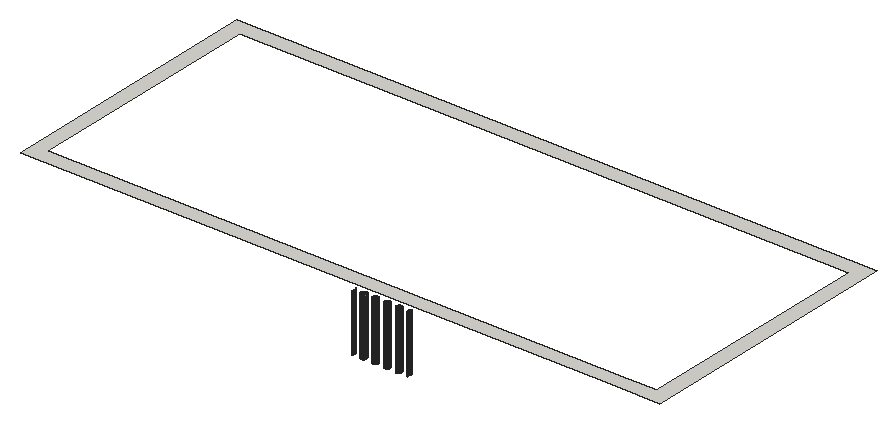
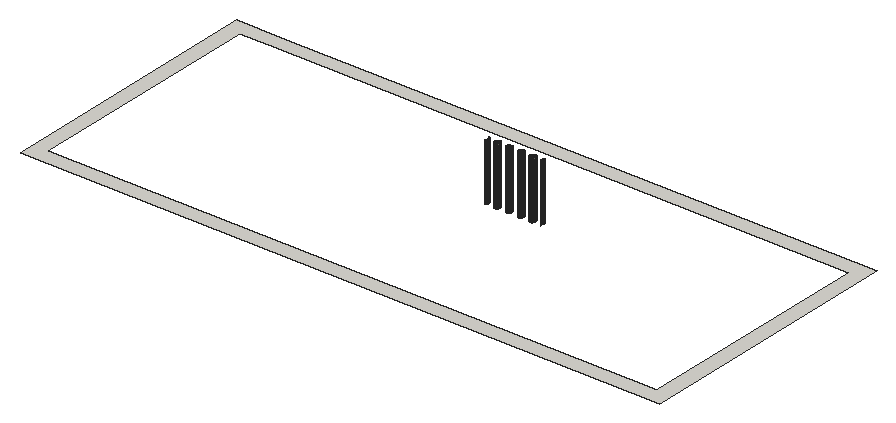
# SketchUp Ruby script. Lengths in inches.
U = 1.inch
M = Sketchup.active_model
def pt(a) = Geom::Point3d.new(a.map { |v| v * U })
def face(e, loops, mat)
  f = e.add_face(loops[0].map { |a| pt(a) })
  loops[1..].each { |l| e.add_face(l.map { |a| pt(a) }).erase! }
  f.material = f.back_material = mat if mat
  f
end
# faces: each face lists its corners as indices into pts; further lists are holes
def faces(e, pts, list, mat = nil) = list.each { |f| face(e, (f[0].is_a?(Array) ? f : [f]).map { |l| l.map { |i| pts[i] } }, mat) }
# xy, xz, yz: faces in a plane at the given z, y or x. An outline is a flat list of corners, or four numbers for a rectangle; further outlines are holes
def ring(l) = l.size == 4 ? [[l[0], l[1]], [l[2], l[1]], [l[2], l[3]], [l[0], l[3]]] : l.each_slice(2).to_a
def flat(e, list, mat, &to3) = list.each { |f| face(e, (f[0].is_a?(Array) ? f : [f]).map { |l| ring(l).map { |u, v| to3.(u, v) } }, mat) }
def xy(e, z, list, mat = nil) = flat(e, list, mat) { |x, y| [x, y, z] }
def xz(e, y, list, mat = nil) = flat(e, list, mat) { |x, z| [x, y, z] }
def yz(e, x, list, mat = nil) = flat(e, list, mat) { |y, z| [x, y, z] }
def lines(e, pts, list) = list.each { |a, b| e.add_line(pt(pts[a]), pt(pts[b])) }
# prism: a flat outline (further loops are holes) pulled along v
def prism(e, loops, v, mat = nil)
  f = face(e, loops, mat); d = Geom::Vector3d.new(v.map { |x| x * U })
  f.pushpull(f.normal.samedirection?(d) ? d.length : -d.length)
end
def box(e, o, s, mat = nil) = prism(e, [[o, [o[0] + s[0], o[1], o[2]], [o[0] + s[0], o[1] + s[1], o[2]], [o[0], o[1] + s[1], o[2]]]], [0, 0, s[2]], mat)
def at(x, y, z, deg = 0) = Geom::Transformation.translation(pt([x, y, z])) * Geom::Transformation.rotation(ORIGIN, Z_AXIS, deg.degrees)
def axes(o, x, y, z) = Geom::Transformation.new([*x, 0, *y, 0, *z, 0, *pt(o).to_a, 1])
def part(name) = M.definitions.add(name)
# library, detail: a bought-in or finely detailed component or shape, given as its bounding box
def library(name, o, s) = part(name).tap { |d| box(d.entities, o, s) }
def detail(e, o, s) = box(e.add_group.entities, o, s)
def put(e, d, t, mat = nil) = e.add_instance(d, t).tap { |i| i.material = mat if mat }
def group(e, t, mat = nil) = e.add_group.tap { |g| g.transformation = t; g.material = mat if mat }.entities
root = M.entities
M.materials.add("[Formica Graystone]").color = [149, 146, 135]
M.materials.add("[Terrazzo Tile Light]").color = [219, 217, 210]
xy(root,552.75,[[326.25,21.93,325.54,22.02,324.875,22.3,324.31,22.74,323.87,23.3,323.59,23.97,323.5,24.68,323.59,25.39,323.87,26.05,324.31,26.625,324.875,27.0625,325.54,27.34,326.25,27.43,326.96,27.34,327.625,27.0625,328.19,26.625,328.63,26.05,328.91,25.39,329,24.68,328.91,23.97,328.63,23.3,328.19,22.74,327.625,22.3,326.96,22.02],[337.625,21.93,336.91,22.02,336.25,22.3,335.68,22.74,335.24,23.3,334.97,23.97,334.875,24.68,334.97,25.39,335.24,26.05,335.68,26.625,336.25,27.0625,336.91,27.34,337.625,27.43,338.34,27.34,339,27.0625,339.57,26.625,340.01,26.05,340.28,25.39,340.375,24.68,340.28,23.97,340.01,23.3,339.57,22.74,339,22.3,338.34,22.02],[349,21.93,348.29,22.02,347.625,22.3,347.06,22.74,346.62,23.3,346.34,23.97,346.25,24.68,346.34,25.39,346.62,26.05,347.06,26.625,347.625,27.0625,348.29,27.34,349,27.43,349.71,27.34,350.375,27.0625,350.94,26.625,351.38,26.05,351.66,25.39,351.75,24.68,351.66,23.97,351.38,23.3,350.94,22.74,350.375,22.3,349.71,22.02],[360.375,21.93,359.66,22.02,359,22.3,358.43,22.74,357.99,23.3,357.72,23.97,357.625,24.68,357.72,25.39,357.99,26.05,358.43,26.625,359,27.0625,359.66,27.34,360.375,27.43,361.09,27.34,361.75,27.0625,362.32,26.625,362.76,26.05,363.03,25.39,363.125,24.68,363.03,23.97,362.76,23.3,362.32,22.74,361.75,22.3,361.09,22.02]])
xy(root,619.9375,[[0,16.1875,577.38,16.1875,577.38,31.11,14.92,31.11,14.92,263.56,605.2,263.56,605.2,31.11,577.38,31.11,577.38,16.1875,620.12,16.1875,620.12,278.48,0,278.48]],"[Terrazzo Tile Light]")
p = [[325.54,22.02,552.75],[326.25,21.93,552.75],[326.25,21.93,608.75],[325.54,22.02,608.75],[326.96,22.02,552.75],[326.96,22.02,608.75],
  [336.91,22.02,552.75],[337.625,21.93,552.75],[337.625,21.93,608.75],[336.91,22.02,608.75],[338.34,22.02,552.75],[338.34,22.02,608.75],
  [348.29,22.02,552.75],[349,21.93,552.75],[349,21.93,608.75],[348.29,22.02,608.75],[349.71,22.02,552.75],[349.71,22.02,608.75],
  [359.66,22.02,552.75],[360.375,21.93,552.75],[360.375,21.93,608.75],[359.66,22.02,608.75],[361.09,22.02,552.75],[361.09,22.02,608.75],
  [324.875,22.3,552.75],[324.875,22.3,608.75],[327.625,22.3,552.75],[327.625,22.3,608.75],[336.25,22.3,552.75],[336.25,22.3,608.75],
  [339,22.3,552.75],[339,22.3,608.75],[347.625,22.3,552.75],[347.625,22.3,608.75],[350.375,22.3,552.75],[350.375,22.3,608.75],
  [359,22.3,552.75],[359,22.3,608.75],[361.75,22.3,552.75],[361.75,22.3,608.75],[370.375,22.3,552.75],[371.04,22.02,552.75],
  [371.04,22.02,608.75],[370.375,22.3,608.75],[316.25,22.3,552.75],[316.82,22.74,552.75],[316.82,22.74,608.75],[316.25,22.3,608.75],
  [324.31,22.74,552.75],[324.31,22.74,608.75],[328.19,22.74,552.75],[328.19,22.74,608.75],[335.68,22.74,552.75],[335.68,22.74,608.75],
  [339.57,22.74,552.75],[339.57,22.74,608.75],[347.06,22.74,552.75],[347.06,22.74,608.75],[350.94,22.74,552.75],[350.94,22.74,608.75],
  [358.43,22.74,552.75],[358.43,22.74,608.75],[362.32,22.74,552.75],[362.32,22.74,608.75],[369.81,22.74,552.75],[369.81,22.74,608.75],
  [317.26,23.3,552.75],[317.26,23.3,608.75],[323.87,23.3,552.75],[323.87,23.3,608.75],[328.63,23.3,552.75],[328.63,23.3,608.75],
  [335.24,23.3,552.75],[335.24,23.3,608.75],[340.01,23.3,552.75],[340.01,23.3,608.75],[346.62,23.3,552.75],[346.62,23.3,608.75],
  [351.38,23.3,552.75],[351.38,23.3,608.75],[357.99,23.3,552.75],[357.99,23.3,608.75],[362.76,23.3,552.75],[362.76,23.3,608.75],
  [369.37,23.3,552.75],[369.37,23.3,608.75],[317.53,23.97,552.75],[317.53,23.97,608.75],[323.59,23.97,552.75],[323.59,23.97,608.75],
  [328.91,23.97,552.75],[328.91,23.97,608.75],[334.97,23.97,552.75],[334.97,23.97,608.75],[340.28,23.97,552.75],[340.28,23.97,608.75],
  [346.34,23.97,552.75],[346.34,23.97,608.75],[351.66,23.97,552.75],[351.66,23.97,608.75],[357.72,23.97,552.75],[357.72,23.97,608.75],
  [363.03,23.97,552.75],[363.03,23.97,608.75],[369.09,23.97,552.75],[369.09,23.97,608.75],[317.625,24.68,552.75],[317.625,24.68,608.75],
  [323.5,24.68,552.75],[323.5,24.68,608.75],[329,24.68,552.75],[329,24.68,608.75],[334.875,24.68,552.75],[334.875,24.68,608.75],
  [340.375,24.68,552.75],[340.375,24.68,608.75],[346.25,24.68,552.75],[346.25,24.68,608.75],[351.75,24.68,552.75],[351.75,24.68,608.75],
  [357.625,24.68,552.75],[357.625,24.68,608.75],[363.125,24.68,552.75],[363.125,24.68,608.75],[369,24.68,552.75],[369,24.68,608.75],
  [317.53,25.39,552.75],[317.53,25.39,608.75],[323.59,25.39,552.75],[323.59,25.39,608.75],[328.91,25.39,552.75],[328.91,25.39,608.75],
  [334.97,25.39,552.75],[334.97,25.39,608.75],[340.28,25.39,552.75],[340.28,25.39,608.75],[346.34,25.39,552.75],[346.34,25.39,608.75],
  [351.66,25.39,552.75],[351.66,25.39,608.75],[357.72,25.39,552.75],[357.72,25.39,608.75],[363.03,25.39,552.75],[363.03,25.39,608.75],
  [369.09,25.39,552.75],[369.09,25.39,608.75],[317.26,26.05,552.75],[317.26,26.05,608.75],[323.87,26.05,552.75],[323.87,26.05,608.75],
  [328.63,26.05,552.75],[328.63,26.05,608.75],[335.24,26.05,552.75],[335.24,26.05,608.75],[340.01,26.05,552.75],[340.01,26.05,608.75],
  [346.62,26.05,552.75],[346.62,26.05,608.75],[351.38,26.05,552.75],[351.38,26.05,608.75],[357.99,26.05,552.75],[357.99,26.05,608.75],
  [362.76,26.05,552.75],[362.76,26.05,608.75],[369.37,26.05,552.75],[369.37,26.05,608.75],[316.82,26.625,552.75],[316.82,26.625,608.75],
  [324.31,26.625,552.75],[324.31,26.625,608.75],[328.19,26.625,552.75],[328.19,26.625,608.75],[335.68,26.625,552.75],[335.68,26.625,608.75],
  [339.57,26.625,552.75],[339.57,26.625,608.75],[347.06,26.625,552.75],[347.06,26.625,608.75],[350.94,26.625,552.75],[350.94,26.625,608.75],
  [358.43,26.625,552.75],[358.43,26.625,608.75],[362.32,26.625,552.75],[362.32,26.625,608.75],[369.81,26.625,552.75],[369.81,26.625,608.75],
  [316.25,27.0625,552.75],[316.25,27.0625,608.75],[324.875,27.0625,552.75],[324.875,27.0625,608.75],[327.625,27.0625,552.75],[327.625,27.0625,608.75],
  [336.25,27.0625,552.75],[336.25,27.0625,608.75],[339,27.0625,552.75],[339,27.0625,608.75],[347.625,27.0625,552.75],[347.625,27.0625,608.75],
  [350.375,27.0625,552.75],[350.375,27.0625,608.75],[359,27.0625,552.75],[359,27.0625,608.75],[361.75,27.0625,552.75],[361.75,27.0625,608.75],
  [370.375,27.0625,552.75],[370.375,27.0625,608.75],[325.54,27.34,552.75],[325.54,27.34,608.75],[326.96,27.34,552.75],[326.96,27.34,608.75],
  [336.91,27.34,552.75],[336.91,27.34,608.75],[338.34,27.34,552.75],[338.34,27.34,608.75],[348.29,27.34,552.75],[348.29,27.34,608.75],
  [349.71,27.34,552.75],[349.71,27.34,608.75],[359.66,27.34,552.75],[359.66,27.34,608.75],[361.09,27.34,552.75],[361.09,27.34,608.75],
  [371.04,27.34,552.75],[371.04,27.34,608.75],[326.25,27.43,552.75],[326.25,27.43,608.75],[337.625,27.43,552.75],[337.625,27.43,608.75],
  [349,27.43,552.75],[349,27.43,608.75],[360.375,27.43,552.75],[360.375,27.43,608.75]]
faces(root,p,[[0,1,2,3],[1,4,5,2],[6,7,8,9],[7,10,11,8],[12,13,14,15],[13,16,17,14],[18,19,20,21],[19,22,23,20],
  [24,0,3,25],[4,26,27,5],[28,6,9,29],[10,30,31,11],[32,12,15,33],[16,34,35,17],[36,18,21,37],[22,38,39,23],
  [40,41,42,43],[44,45,46,47],[48,24,25,49],[26,50,51,27],[52,28,29,53],[30,54,55,31],[56,32,33,57],[34,58,59,35],
  [60,36,37,61],[38,62,63,39],[64,40,43,65],[45,66,67,46],[68,48,49,69],[50,70,71,51],[72,52,53,73],[54,74,75,55],
  [76,56,57,77],[58,78,79,59],[80,60,61,81],[62,82,83,63],[84,64,65,85],[66,86,87,67],[88,68,69,89],[70,90,91,71],
  [92,72,73,93],[74,94,95,75],[96,76,77,97],[78,98,99,79],[100,80,81,101],[82,102,103,83],[104,84,85,105],[86,106,107,87],
  [108,88,89,109],[90,110,111,91],[112,92,93,113],[94,114,115,95],[116,96,97,117],[98,118,119,99],[120,100,101,121],[102,122,123,103],
  [124,104,105,125],[106,126,127,107],[128,108,109,129],[110,130,131,111],[132,112,113,133],[114,134,135,115],[136,116,117,137],[118,138,139,119],
  [140,120,121,141],[122,142,143,123],[144,124,125,145],[126,146,147,127],[148,128,129,149],[130,150,151,131],[152,132,133,153],[134,154,155,135],
  [156,136,137,157],[138,158,159,139],[160,140,141,161],[142,162,163,143],[164,144,145,165],[146,166,167,147],[168,148,149,169],[150,170,171,151],
  [172,152,153,173],[154,174,175,155],[176,156,157,177],[158,178,179,159],[180,160,161,181],[162,182,183,163],[184,164,165,185],[166,186,187,167],
  [188,168,169,189],[170,190,191,171],[192,172,173,193],[174,194,195,175],[196,176,177,197],[178,198,199,179],[200,180,181,201],[182,202,203,183],
  [204,184,185,205],[206,188,189,207],[190,208,209,191],[210,192,193,211],[194,212,213,195],[214,196,197,215],[198,216,217,199],[218,200,201,219],
  [202,220,221,203],[222,204,205,223],[224,206,207,225],[208,224,225,209],[226,210,211,227],[212,226,227,213],[228,214,215,229],[216,228,229,217],
  [230,218,219,231],[220,230,231,221]],"[Formica Graystone]")
